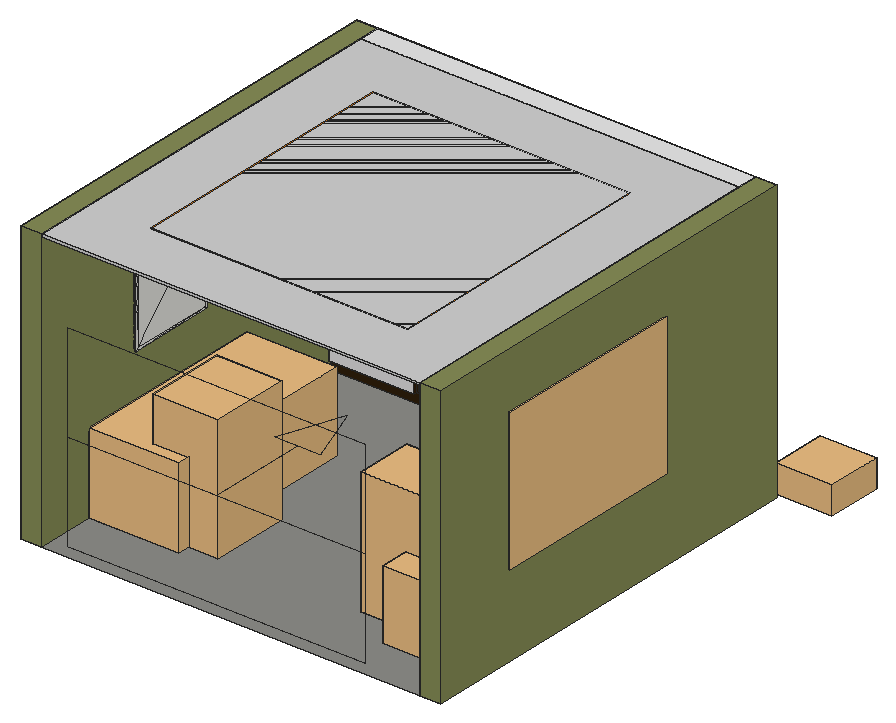
# SketchUp Ruby script. Lengths in inches.
U = 1.inch
M = Sketchup.active_model
def pt(a) = Geom::Point3d.new(a.map { |v| v * U })
def face(e, loops, mat)
  f = e.add_face(loops[0].map { |a| pt(a) })
  loops[1..].each { |l| e.add_face(l.map { |a| pt(a) }).erase! }
  f.material = f.back_material = mat if mat
  f
end
# faces: each face lists its corners as indices into pts; further lists are holes
def faces(e, pts, list, mat = nil) = list.each { |f| face(e, (f[0].is_a?(Array) ? f : [f]).map { |l| l.map { |i| pts[i] } }, mat) }
# xy, xz, yz: faces in a plane at the given z, y or x. An outline is a flat list of corners, or four numbers for a rectangle; further outlines are holes
def ring(l) = l.size == 4 ? [[l[0], l[1]], [l[2], l[1]], [l[2], l[3]], [l[0], l[3]]] : l.each_slice(2).to_a
def flat(e, list, mat, &to3) = list.each { |f| face(e, (f[0].is_a?(Array) ? f : [f]).map { |l| ring(l).map { |u, v| to3.(u, v) } }, mat) }
def xy(e, z, list, mat = nil) = flat(e, list, mat) { |x, y| [x, y, z] }
def xz(e, y, list, mat = nil) = flat(e, list, mat) { |x, z| [x, y, z] }
def yz(e, x, list, mat = nil) = flat(e, list, mat) { |y, z| [x, y, z] }
def lines(e, pts, list) = list.each { |a, b| e.add_line(pt(pts[a]), pt(pts[b])) }
# prism: a flat outline (further loops are holes) pulled along v
def prism(e, loops, v, mat = nil)
  f = face(e, loops, mat); d = Geom::Vector3d.new(v.map { |x| x * U })
  f.pushpull(f.normal.samedirection?(d) ? d.length : -d.length)
end
def box(e, o, s, mat = nil) = prism(e, [[o, [o[0] + s[0], o[1], o[2]], [o[0] + s[0], o[1] + s[1], o[2]], [o[0], o[1] + s[1], o[2]]]], [0, 0, s[2]], mat)
def at(x, y, z, deg = 0) = Geom::Transformation.translation(pt([x, y, z])) * Geom::Transformation.rotation(ORIGIN, Z_AXIS, deg.degrees)
def axes(o, x, y, z) = Geom::Transformation.new([*x, 0, *y, 0, *z, 0, *pt(o).to_a, 1])
def part(name) = M.definitions.add(name)
# library, detail: a bought-in or finely detailed component or shape, given as its bounding box
def library(name, o, s) = part(name).tap { |d| box(d.entities, o, s) }
def detail(e, o, s) = box(e.add_group.entities, o, s)
def put(e, d, t, mat = nil) = e.add_instance(d, t).tap { |i| i.material = mat if mat }
def group(e, t, mat = nil) = e.add_group.tap { |g| g.transformation = t; g.material = mat if mat }.entities
root = M.entities
M.materials.add("Emissive").color = [255, 146, 33]
M.materials.add("Emissive\#1").color = [255, 146, 33]
M.materials.add("Marble White 23-73 150cm").color = [221, 220, 222]
M.materials.add("Marble White SSS 100cm").color = [222, 222, 222]
M.materials.add("Tiles Grey 13 135cm").color = [141, 141, 136]
M.materials.add("Wall Paint Fine Grain 01 White 100cm").color = [208, 208, 208]
M.materials.add("Wall Paint Olive Matte 300cm").color = [133, 140, 86]
M.materials.add("Wall Paint White Semigloss 300cm").color = [232, 232, 232]
M.materials.add("Wood Walnut 33-38 100cm").color = [48, 31, 12]
c1 = library("Rue De Babylone Sofa",[-49.17,-15.95,0],[98.34,31.9,29.73])
c2 = library("Vera Sofa with Skirt",[-42.23,-17.43,0],[84.46,38.26,34.375])
c3 = library("Books 284 012",[-3.9,-5.03,0],[7.8,10.06,1.71])
c4 = library("Radio 114 011",[-4.52,-2.59,0],[9.04,5.18,10])
c5 = library("Metal Robot 114 042",[-2.05,-1.33,0],[4.11,2.66,7.35])
c6 = library("Interior Props 221 021",[-4.05,-2.74,-0.04],[8.1,5.5,13.08])
c7 = library("Vase 193 006",[-6.57,-6.63,0],[14.76,12.62,17.43])
c8 = library("Magazine 193 001",[-10.16,-7.05,0],[21.59,13.95,2.71])
c9 = library("Vase 004",[-7.23,-6.39,-0.02],[13.74,12.68,17.81])
c10 = library("Router 156 006",[-4.3,-2.49,-0.03],[9,4.96,4.68])
c11 = library("Toy 155 013",[-1.73,-1.4375,0],[3.14,2.99,4.15])
c12 = part("Print Art 008")
xy(c12.entities,-18.54,[[-18.4,-0.29,-18.4,-0.1,18.4,-0.29],[18.4,-0.29,-18.4,-0.1,18.4,-0.1]])
xy(c12.entities,-18.02,[[-18.02,-0.98,18.02,-0.01,-18.02,-0.01],[-18.02,-0.98,18.02,-0.98,18.02,-0.01]])
xy(c12.entities,-18,[[-18,-0.94,-18,-0.45,18,-0.94],[18,-0.94,-18,-0.45,18,-0.45]])
xy(c12.entities,18,[[-18,-0.94,18,-0.45,-18,-0.45],[-18,-0.94,18,-0.94,18,-0.45]])
xy(c12.entities,18.02,[[-18.02,-0.98,-18.02,-0.01,18.02,-0.98],[18.02,-0.98,-18.02,-0.01,18.02,-0.01]])
xy(c12.entities,18.54,[[-18.4,-0.29,18.4,-0.1,-18.4,-0.1],[-18.4,-0.29,18.4,-0.29,18.4,-0.1]])
xz(c12.entities,-0.98,[[-18.99,-18.99,-18.02,-18.02,-18.99,18.99],[-18.99,-18.99,18.02,-18.02,-18.02,-18.02],[-18.99,-18.99,18.99,-18.99,18.02,-18.02],[18.99,-18.99,18.02,18.02,18.02,-18.02],[18.99,-18.99,18.99,18.99,18.02,18.02],
  [-18.02,-18.02,-18.02,18.02,-18.99,18.99],[-18.02,18.02,18.99,18.99,-18.99,18.99],[-18.02,18.02,18.02,18.02,18.99,18.99]])
xz(c12.entities,-0.94,[[-18,-18,18,-18,18,18],[-18,-18,18,18,-18,18]])
xz(c12.entities,-0.45,[[-18,-18,-18,18,18,18],[-18,-18,18,18,18,-18]])
xz(c12.entities,-0.29,[[-18.4,-18.54,18.4,-18.54,18.4,18.54],[-18.4,-18.54,18.4,18.54,-18.4,18.54]])
xz(c12.entities,-0.1,[[-18.4,-18.54,-18.4,18.54,18.4,18.54],[-18.4,-18.54,18.4,18.54,18.4,-18.54]])
xz(c12.entities,-0.01,[[-18.98,-18.98,-18.02,-18.02,18.98,-18.98],[-18.98,-18.98,-18.02,18.02,-18.02,-18.02],[-18.98,-18.98,-18.98,18.98,-18.02,18.02],[18.98,-18.98,-18.02,-18.02,18.02,-18.02],[18.98,-18.98,18.02,-18.02,18.98,18.98],
  [18.02,-18.02,18.02,18.02,18.98,18.98],[-18.02,18.02,-18.98,18.98,18.02,18.02],[18.02,18.02,-18.98,18.98,18.98,18.98]])
yz(c12.entities,-18.4,[[-0.29,-18.54,-0.1,18.54,-0.1,-18.54],[-0.29,-18.54,-0.29,18.54,-0.1,18.54]])
yz(c12.entities,-18.02,[[-0.01,-18.02,-0.01,18.02,-0.98,18.02],[-0.98,-18.02,-0.01,-18.02,-0.98,18.02]])
yz(c12.entities,-18,[[-0.94,-18,-0.45,18,-0.45,-18],[-0.94,-18,-0.94,18,-0.45,18]])
yz(c12.entities,18,[[-0.45,-18,-0.45,18,-0.94,18],[-0.94,-18,-0.45,-18,-0.94,18]])
yz(c12.entities,18.02,[[-0.98,-18.02,-0.01,18.02,-0.01,-18.02],[-0.98,-18.02,-0.98,18.02,-0.01,18.02]])
yz(c12.entities,18.4,[[-0.1,-18.54,-0.1,18.54,-0.29,18.54],[-0.29,-18.54,-0.1,-18.54,-0.29,18.54]])
p = [[-18.98,-0.01,18.98],[-18.98,-0.01,-18.98],[-18.99,-0.98,-18.99],[-18.99,-0.98,18.99],[18.98,-0.01,-18.98],[18.99,-0.98,-18.99],
  [18.98,-0.01,18.98],[18.99,-0.98,18.99]]
faces(c12.entities,p,[[0,1,2],[2,3,0],[1,4,5],[5,2,1],[4,6,7],[7,5,4],[6,0,3],[3,7,6]])
c13 = library("Air Conditioner 12-08",[-17.72,-4.75,-0.8125],[35.44,4.75,9.47])
c14 = library("Johnny Sitting 001",[-16.98,-13.88,0],[33.96,27.76,53.26])
c15 = library("Jerald Sitting 001",[-12.16,-14.11,0],[24.32,28.22,53.59])
c16 = part("Group37\#1")
p = [[0,0,0],[0,0,-6.8],[-2.75,0,-6.8],[17.875,-4.15,0],[-17.875,-4.15,0],[17.875,4.15,0],
  [17.875,0,0],[-17.875,4.15,0],[2.75,0,-6.8],[-17.875,0,0],[0,0,-11.01]]
lines(c16.entities,p,[[0,1],[1,2],[3,4],[5,6],[7,5],[1,8],[9,0],[0,6],[8,10],[4,9],[6,3],[2,10],
  [9,7]])
c17 = part("Rectangle Light")
put(c17.entities,c16,at(0,0,0))
c18 = library("IES Light",[-4.45,-4.45,-12],[8.9,8.9,12])
c19 = library("Dome Light",[-12,-12,0],[24,24,12])
c20 = part("Group45\#1")
p = [[0,0,0],[0,0,-43.4],[-12.44,0,-43.4],[81,-59.5,0],[-81,-59.5,0],[81,59.5,0],
  [81,0,0],[-81,59.5,0],[12.44,0,-43.4],[-81,0,0],[0,0,-70.25]]
lines(c20.entities,p,[[0,1],[1,2],[3,4],[5,6],[7,5],[1,8],[9,0],[0,6],[8,10],[4,9],[6,3],[2,10],
  [9,7]])
c21 = part("Rectangle Light\#1")
put(c21.entities,c20,at(0,0,0))
c22 = library("Curtains 47-25 merged",[-45.98,-3.97,-0.23],[91.96,10.81,94.58])
c23 = library("Window 46-08 merged",[-34.875,-3.16,0],[69.74,4.26,70.87])
c24 = library("TV 156 039 merged",[-24.43,-3.69,-0.14],[48.87,7.6,29.26])
c25 = part("Vertical wall slat")
xy(c25.entities,-47.05,[[195.61,-2,197.61,0]])
xy(c25.entities,60.95,[[195.61,-2,197.61,0]])
xz(c25.entities,-2,[[195.61,-47.05,197.61,60.95]],"Wood Walnut 33-38 100cm")
xz(c25.entities,0,[[195.61,-47.05,197.61,60.95]])
yz(c25.entities,195.61,[[-2,-47.05,0,60.95]])
yz(c25.entities,197.61,[[-2,-47.05,0,60.95]],"Wood Walnut 33-38 100cm")
c26 = library("IES Light\#1",[-4.45,-4.45,-12],[8.9,8.9,12])
c27 = part("Recessed downlight")
xy(c27.entities,-1,[[3,1,3.52,1.07,4,1.27,4.41,1.59,4.73,2,4.93,2.48,5,3,4.93,3.52,4.73,4,4.41,4.41,4,4.73,3.52,4.93,3,5,2.48,4.93,2,4.73,1.59,4.41,1.27,4,1.07,3.52,1,3,1.07,2.48,1.27,2,1.59,1.59,2,1.27,2.48,1.07]])
xy(c27.entities,0,[[[3,0,2.22,0.1,1.5,0.4,0.88,0.88,0.4,1.5,0.1,2.22,0,3,0.1,3.78,0.4,4.5,0.88,5.12,1.5,5.6,2.22,5.9,3,6,3.78,5.9,4.5,5.6,5.12,5.12,5.6,4.5,5.9,3.78,6,3,5.9,2.22,5.6,1.5,5.12,0.88,4.5,0.4,3.78,0.1],[3,1,3.52,1.07,4,1.27,4.41,1.59,4.73,2,4.93,2.48,5,3,4.93,3.52,4.73,4,4.41,4.41,4,4.73,3.52,4.93,3,5,2.48,4.93,2,4.73,1.59,4.41,1.27,4,1.07,3.52,1,3,1.07,2.48,1.27,2,1.59,1.59,2,1.27,2.48,1.07]]])
xy(c27.entities,0.5,[[[3,0,3.78,0.1,4.5,0.4,5.12,0.88,5.6,1.5,5.9,2.22,6,3,5.9,3.78,5.6,4.5,5.12,5.12,4.5,5.6,3.78,5.9,3,6,2.22,5.9,1.5,5.6,0.88,5.12,0.4,4.5,0.1,3.78,0,3,0.1,2.22,0.4,1.5,0.88,0.88,1.5,0.4,2.22,0.1],[3,1,2.48,1.07,2,1.27,1.59,1.59,1.27,2,1.07,2.48,1,3,1.07,3.52,1.27,4,1.59,4.41,2,4.73,2.48,4.93,3,5,3.52,4.93,4,4.73,4.41,4.41,4.73,4,4.93,3.52,5,3,4.93,2.48,4.73,2,4.41,1.59,4,1.27,3.52,1.07]]])
p = [[2.48,1.07,-1],[2.48,1.07,0],[2.48,1.07,0.5],[3,1,0.5],[3,1,0],[3,1,-1],
  [3.52,1.07,0.5],[3.52,1.07,0],[3.52,1.07,-1],[2,1.27,-1],[2,1.27,0],[2,1.27,0.5],
  [4,1.27,0.5],[4,1.27,0],[4,1.27,-1],[1.59,1.59,-1],[1.59,1.59,0],[1.59,1.59,0.5],
  [4.41,1.59,0.5],[4.41,1.59,0],[4.41,1.59,-1],[1.27,2,-1],[1.27,2,0],[1.27,2,0.5],
  [4.73,2,0.5],[4.73,2,0],[4.73,2,-1],[1.07,2.48,-1],[1.07,2.48,0],[1.07,2.48,0.5],
  [4.93,2.48,0.5],[4.93,2.48,0],[4.93,2.48,-1],[1,3,-1],[1,3,0],[1,3,0.5],
  [5,3,0.5],[5,3,0],[5,3,-1],[1.07,3.52,-1],[1.07,3.52,0],[1.07,3.52,0.5],
  [4.93,3.52,0.5],[4.93,3.52,0],[4.93,3.52,-1],[1.27,4,-1],[1.27,4,0],[1.27,4,0.5],
  [4.73,4,0.5],[4.73,4,0],[4.73,4,-1],[1.59,4.41,-1],[1.59,4.41,0],[1.59,4.41,0.5],
  [4.41,4.41,0.5],[4.41,4.41,0],[4.41,4.41,-1],[2,4.73,-1],[2,4.73,0],[2,4.73,0.5],
  [4,4.73,0.5],[4,4.73,0],[4,4.73,-1],[2.48,4.93,-1],[2.48,4.93,0],[2.48,4.93,0.5],
  [3.52,4.93,0.5],[3.52,4.93,0],[3.52,4.93,-1],[3,5,-1],[3,5,0],[3,5,0.5],
  [2.22,0.1,0],[3,0,0],[3,0,0.5],[2.22,0.1,0.5],[3.78,0.1,0],[3.78,0.1,0.5],
  [1.5,0.4,0],[1.5,0.4,0.5],[4.5,0.4,0],[4.5,0.4,0.5],[0.88,0.88,0],[0.88,0.88,0.5],
  [5.12,0.88,0],[5.12,0.88,0.5],[0.4,1.5,0],[0.4,1.5,0.5],[5.6,1.5,0],[5.6,1.5,0.5],
  [0.1,2.22,0],[0.1,2.22,0.5],[5.9,2.22,0],[5.9,2.22,0.5],[0,3,0],[0,3,0.5],
  [6,3,0],[6,3,0.5],[0.1,3.78,0],[0.1,3.78,0.5],[5.9,3.78,0],[5.9,3.78,0.5],
  [0.4,4.5,0],[0.4,4.5,0.5],[5.6,4.5,0],[5.6,4.5,0.5],[0.88,5.12,0],[0.88,5.12,0.5],
  [5.12,5.12,0],[5.12,5.12,0.5],[1.5,5.6,0],[1.5,5.6,0.5],[4.5,5.6,0],[4.5,5.6,0.5],
  [2.22,5.9,0],[2.22,5.9,0.5],[3.78,5.9,0],[3.78,5.9,0.5],[3,6,0],[3,6,0.5]]
faces(c27.entities,p,[[0,1,2,3,4,5],[5,4,3,6,7,8],[9,10,11,2,1,0],[8,7,6,12,13,14],[15,16,17,11,10,9],[14,13,12,18,19,20],[21,22,23,17,16,15],[20,19,18,24,25,26],
  [27,28,29,23,22,21],[26,25,24,30,31,32],[33,34,35,29,28,27],[32,31,30,36,37,38],[39,40,41,35,34,33],[38,37,36,42,43,44],[45,46,47,41,40,39],[44,43,42,48,49,50],
  [51,52,53,47,46,45],[50,49,48,54,55,56],[57,58,59,53,52,51],[56,55,54,60,61,62],[63,64,65,59,58,57],[62,61,60,66,67,68],[69,70,71,65,64,63],[68,67,66,71,70,69],
  [72,73,74,75],[73,76,77,74],[78,72,75,79],[76,80,81,77],[82,78,79,83],[80,84,85,81],[86,82,83,87],[84,88,89,85],
  [90,86,87,91],[88,92,93,89],[94,90,91,95],[92,96,97,93],[98,94,95,99],[96,100,101,97],[102,98,99,103],[100,104,105,101],
  [106,102,103,107],[104,108,109,105],[110,106,107,111],[108,112,113,109],[114,110,111,115],[112,116,117,113],[118,114,115,119],[116,118,119,117]])
put(c27.entities,c26,axes([3,3,0.76],[1,0,0],[0,1,0],[0,0,-1]))
xy(root,47.32,[[61.2,168.17,60.93,168.26,61.48,168.22],[82.18,168.17,81.91,168.26,82.46,168.22],[61.48,168.22,60.93,168.26,61.78,168.68],[61.48,168.22,61.78,168.68,61.69,168.41],[82.46,168.22,81.91,168.26,82.76,168.68],
  [82.46,168.22,82.76,168.68,82.67,168.41],[60.93,168.26,60.69,168.75,60.99,169.21],[60.93,168.26,60.74,168.47,60.69,168.75],[60.93,168.26,60.99,169.21,61.78,168.68],[81.91,168.26,81.66,168.75,81.97,169.21],
  [81.91,168.26,81.72,168.47,81.66,168.75],[81.91,168.26,81.97,169.21,82.76,168.68],[61.78,168.68,60.99,169.21,61.54,169.17],[61.78,168.68,61.54,169.17,61.73,168.96],[82.76,168.68,81.97,169.21,82.52,169.17],
  [82.76,168.68,82.52,169.17,82.71,168.96],[60.69,168.75,60.78,169.02,60.99,169.21],[81.66,168.75,81.76,169.02,81.97,169.21],[61.54,169.17,60.99,169.21,61.27,169.26],[82.52,169.17,81.97,169.21,82.25,169.26]])
xy(root,47.36,[[61.2,168.17,61.48,168.22,60.93,168.26],[82.18,168.17,82.46,168.22,81.91,168.26],[61.48,168.22,60.69,168.75,60.93,168.26],[61.48,168.22,61.54,169.17,60.69,168.75],[61.48,168.22,61.69,168.41,61.78,168.68],
  [61.48,168.22,61.78,168.68,61.54,169.17],[82.46,168.22,81.66,168.75,81.91,168.26],[82.46,168.22,82.52,169.17,81.66,168.75],[82.46,168.22,82.67,168.41,82.76,168.68],[82.46,168.22,82.76,168.68,82.52,169.17],
  [60.93,168.26,60.69,168.75,60.74,168.47],[81.91,168.26,81.66,168.75,81.72,168.47],[61.78,168.68,61.73,168.96,61.54,169.17],[82.76,168.68,82.71,168.96,82.52,169.17],[60.69,168.75,60.99,169.21,60.78,169.02],
  [60.69,168.75,61.54,169.17,60.99,169.21],[81.66,168.75,81.97,169.21,81.76,169.02],[81.66,168.75,82.52,169.17,81.97,169.21],[61.54,169.17,61.27,169.26,60.99,169.21],[82.52,169.17,82.25,169.26,81.97,169.21]])
p = [[61.2,168.17,47.36],[60.93,168.26,47.36],[60.93,168.26,47.32],[61.2,168.17,47.32],[61.48,168.22,47.36],[61.48,168.22,47.32],
  [61.69,168.41,47.36],[61.69,168.41,47.32],[82.18,168.17,47.36],[81.91,168.26,47.36],[81.91,168.26,47.32],[82.18,168.17,47.32],
  [82.46,168.22,47.36],[82.46,168.22,47.32],[82.67,168.41,47.36],[82.67,168.41,47.32],[60.74,168.47,47.36],[60.74,168.47,47.32],
  [81.72,168.47,47.36],[81.72,168.47,47.32],[61.78,168.68,47.36],[61.78,168.68,47.32],[82.76,168.68,47.36],[82.76,168.68,47.32],
  [60.69,168.75,47.36],[60.69,168.75,47.32],[81.66,168.75,47.36],[81.66,168.75,47.32],[61.73,168.96,47.36],[61.73,168.96,47.32],
  [82.71,168.96,47.36],[82.71,168.96,47.32],[60.78,169.02,47.36],[60.78,169.02,47.32],[81.76,169.02,47.36],[81.76,169.02,47.32],
  [60.99,169.21,47.36],[60.99,169.21,47.32],[61.54,169.17,47.36],[61.54,169.17,47.32],[81.97,169.21,47.36],[81.97,169.21,47.32],
  [82.52,169.17,47.36],[82.52,169.17,47.32],[61.27,169.26,47.36],[61.27,169.26,47.32],[82.25,169.26,47.36],[82.25,169.26,47.32]]
faces(root,p,[[0,1,2],[2,3,0],[4,0,3],[3,5,4],[6,4,5],[5,7,6],[8,9,10],[10,11,8],
  [12,8,11],[11,13,12],[14,12,13],[13,15,14],[1,16,17],[17,2,1],[9,18,19],[19,10,9],
  [20,6,7],[7,21,20],[22,14,15],[15,23,22],[16,24,25],[25,17,16],[18,26,27],[27,19,18],
  [28,20,21],[21,29,28],[30,22,23],[23,31,30],[24,32,33],[33,25,24],[26,34,35],[35,27,26],
  [32,36,37],[37,33,32],[38,28,29],[29,39,38],[34,40,41],[41,35,34],[42,30,31],[31,43,42],
  [36,44,45],[45,37,36],[44,38,39],[39,45,44],[40,46,47],[47,41,40],[46,42,43],[43,47,46]])
put(root,c1,axes([155.05,69.1875,0],[0,1,0],[1,0,0],[0,0,1]))
put(root,c2,at(29.83,67.89,0,90))
put(root,c3,at(100.82,160.36,10))
put(root,c3,at(18.98,161.07,16))
put(root,c3,at(164.75,160.875,88.65))
put(root,c4,at(165.17,161.59,18.67))
put(root,c4,at(112.48,159.44,16))
put(root,c5,at(164.75,157,54.32))
put(root,c5,at(28.22,159,16))
put(root,c6,at(153.25,159.74,79.57))
put(root,c6,at(101.77,159.46,16))
put(root,c7,at(63.52,161.36,16))
put(root,c8,at(151.35,99.1,15.21))
put(root,c8,at(35.08,89.79,19.11))
put(root,c9,axes([153.52,163.39,53.02],[0.76413,0,0],[0,1,0],[0,0,1]))
put(root,c9,axes([153.52,160.4375,27.27],[0.76413,0,0],[0,1,0],[0,0,1]))
put(root,c9,axes([153.52,159,1.35],[0.76413,0,0],[0,1,0],[0,0,1]))
put(root,c3,at(164.92,162.66,35.79))
put(root,c10,at(43.27,160.02,16))
put(root,c11,at(164.87,159.84,70.17))
put(root,c12,at(8.99,68.5625,72.53,90))
put(root,c13,at(9,116.47,87.12,90))
put(root,c14,at(46.07,47.85,0,90))
put(root,c15,at(134.01,44.68,0,-90))
put(root,c17,axes([27.75,159.85,14.49],[1,0,0],[0,-1,0],[0,0,0.36]))
put(root,c17,axes([65.84,159.85,14.49],[1,0,0],[0,-1,0],[0,0,0.36]))
put(root,c17,axes([103.33,159.85,14.49],[0.89884,0,0],[0,-1,0],[0,0,0.36]))
put(root,c17,axes([63,161.85,8.25],[0.8633,0,0],[0,-1,0],[0,0,0.22453]))
put(root,c18,axes([153.25,162.05,103.49],[1,0,0],[0,1,0],[0,0,0.78]))
put(root,c18,axes([164.91,162.05,103.49],[1,0,0],[0,1,0],[0,0,0.78]))
put(root,c18,axes([164.91,162.05,85.5625],[1,0,0],[0,1,0],[0,0,0.78]))
put(root,c18,axes([164.91,162.05,67.81],[1,0,0],[0,1,0],[0,0,0.78]))
put(root,c18,axes([153.25,162.05,76.89],[1,0,0],[0,1,0],[0,0,0.78]))
put(root,c18,axes([153.25,162.05,50.99],[1,0,0],[0,1,0],[0,0,0.78]))
put(root,c18,axes([153.25,162.05,25.07],[1,0,0],[0,1,0],[0,0,0.78]))
put(root,c18,axes([164.91,162.05,50.4],[1,0,0],[0,1,0],[0,0,0.78]))
put(root,c18,axes([164.91,162.05,32.99],[1,0,0],[0,1,0],[0,0,0.78]))
put(root,c18,axes([164.91,162.05,15.58],[1,0,0],[0,1,0],[0,0,0.78]))
put(root,c19,at(190.13,193.56,0))
put(root,c21,axes([90.51,-8.13,52.01],[0.7863,0,0],[0,0,-0.70597],[0,-1,0]))
put(root,c22,axes([164.16,79.1,32.65],[0,-1.2932,0],[1,0,0],[0,0,0.7663]))
put(root,c23,axes([176,78,36],[0,1.20437,0],[-1.5872,0,0],[0,0,0.84667]))
put(root,c24,at(73.52,161.09,48.2))
g1 = group(root,at(0,0,0),"Tiles Grey 13 135cm")
xy(g1,0,[[0,0,180,180]],"Tiles Grey 13 135cm")
g2 = group(root,at(0,0,0),"Wall Paint Olive Matte 300cm")
box(g2,[0,0,0],[9,180,120])
g3 = group(root,at(171,0,0),"Wall Paint Olive Matte 300cm")
prism(g3,[[[9,0,0],[9,180,0],[9,180,120],[9,0,120]],[[9,120,96],[9,120,36],[9,36,36],[9,36,96]]],[-9,0,0])
g4 = group(root,at(9,171,0),"Wall Paint White Semigloss 300cm")
box(g4,[0,0,0],[162,9,120])
g5 = group(root,at(9,169,0),"Marble White SSS 100cm")
box(g5,[0,0,0],[162,2,108],"Marble White SSS 100cm")
g6 = group(root,at(147,157,0),"Wood Walnut 33-38 100cm")
xy(g6,0,[[0,0,24,12]],"Wood Walnut 33-38 100cm")
xy(g6,1,[[1,0,11.5,10],[12.5,0,23,10]],"Wood Walnut 33-38 100cm")
xy(g6,17.67,[[12.5,0,23,10]],"Wood Walnut 33-38 100cm")
xy(g6,18.67,[[12.5,0,23,10]],"Wood Walnut 33-38 100cm")
xy(g6,26.25,[[1,0,11.5,10]],"Wood Walnut 33-38 100cm")
xy(g6,27.25,[[1,0,11.5,10]],"Wood Walnut 33-38 100cm")
xy(g6,34.83,[[12.5,0,23,10]],"Wood Walnut 33-38 100cm")
xy(g6,35.83,[[12.5,0,23,10]],"Wood Walnut 33-38 100cm")
xy(g6,52,[[1,0,11.5,10],[12.5,0,23,10]],"Wood Walnut 33-38 100cm")
xy(g6,53,[[1,0,11.5,10],[12.5,0,23,10]],"Wood Walnut 33-38 100cm")
xy(g6,69.17,[[12.5,0,23,10]],"Wood Walnut 33-38 100cm")
xy(g6,70.17,[[12.5,0,23,10]],"Wood Walnut 33-38 100cm")
xy(g6,77.75,[[1,0,11.5,10]],"Wood Walnut 33-38 100cm")
xy(g6,78.75,[[1,0,11.5,10]],"Wood Walnut 33-38 100cm")
xy(g6,86.33,[[12.5,0,23,10]],"Wood Walnut 33-38 100cm")
xy(g6,87.33,[[12.5,0,23,10]],"Wood Walnut 33-38 100cm")
xy(g6,104,[[1,0,11.5,10],[12.5,0,23,10]],"Wood Walnut 33-38 100cm")
xy(g6,108,[[0,0,24,12]],"Wood Walnut 33-38 100cm")
xz(g6,0,[[[0,0,24,108],[1,78.75,11.5,104],[1,1,11.5,26.25],[1,53,11.5,77.75],[1,27.25,11.5,52],[12.5,1,23,17.67],[12.5,87.33,23,104],[12.5,70.17,23,86.33],[12.5,35.83,23,52],[12.5,53,23,69.17],[12.5,18.67,23,34.83]]],"Wood Walnut 33-38 100cm")
xz(g6,10,[[1,1,11.5,26.25],[12.5,1,23,17.67],[12.5,18.67,23,34.83],[1,27.25,11.5,52],[12.5,35.83,23,52],
  [1,53,11.5,77.75],[12.5,53,23,69.17],[12.5,70.17,23,86.33],[1,78.75,11.5,104],[12.5,87.33,23,104]],"Wood Walnut 33-38 100cm")
xz(g6,12,[[0,0,24,108]],"Wood Walnut 33-38 100cm")
yz(g6,0,[[0,0,12,108]],"Wood Walnut 33-38 100cm")
yz(g6,1,[[0,1,10,26.25],[0,27.25,10,52],[0,53,10,77.75],[0,78.75,10,104]],"Wood Walnut 33-38 100cm")
yz(g6,11.5,[[0,1,10,26.25],[0,27.25,10,52],[0,53,10,77.75],[0,78.75,10,104]],"Wood Walnut 33-38 100cm")
yz(g6,12.5,[[0,1,10,17.67],[0,18.67,10,34.83],[0,35.83,10,52],[0,53,10,69.17],[0,70.17,10,86.33],
  [0,87.33,10,104]],"Wood Walnut 33-38 100cm")
yz(g6,23,[[0,1,10,17.67],[0,18.67,10,34.83],[0,35.83,10,52],[0,53,10,69.17],[0,70.17,10,86.33],
  [0,87.33,10,104]],"Wood Walnut 33-38 100cm")
yz(g6,24,[[0,0,12,108]],"Wood Walnut 33-38 100cm")
g7 = group(root,at(9,154,0))
xy(g7,0,[[0,1,114,13]],"Wood Walnut 33-38 100cm")
xy(g7,4,[[0,0,36.5,1],[71.5,0,108,1],[0,1,0,13,114,13,114,1,113,1,113,12,108,12,108,1],[108,1,113,12]],"Wood Walnut 33-38 100cm")
xy(g7,5,[[37.5,1,70.5,12]],"Wood Walnut 33-38 100cm")
xy(g7,9,[[37.5,1,38.5,12],[38.5,1,70.5,12]],"Wood Walnut 33-38 100cm")
xy(g7,10,[[0,0,36.5,1],[71.5,0,75.5,1],[75.5,0,76.5,1],[76.5,0,108,1],[0,1,37.5,12],
  [38.5,1,75.5,12],[76.5,1,108,12]],"Wood Walnut 33-38 100cm")
xy(g7,15,[[0,1,37.5,12],[38.5,1,75.5,12],[76.5,1,113,12]],"Wood Walnut 33-38 100cm")
xy(g7,16,[[0,1,114,13]],"Wood Walnut 33-38 100cm")
xz(g7,1,[[0,0,114,4],[0,4,36.5,10],[113,4,114,4,114,16,0,16,0,15,37.5,15,37.5,10,38.5,10,38.5,15,75.5,15,75.5,10,76.5,10,76.5,15,113,15],[[36.5,4,71.5,10],[37.5,5,70.5,9]],[71.5,4,108,10]],"Wood Walnut 33-38 100cm")
xz(g7,12,[[108,4,113,4,113,15,76.5,15,76.5,10,108,10],[37.5,5,70.5,9],[0,10,37.5,15],[38.5,10,75.5,15]],"Wood Walnut 33-38 100cm")
xz(g7,13,[[0,0,114,4],[0,4,114,10],[0,10,114,16]],"Wood Walnut 33-38 100cm")
yz(g7,0,[[1,0,13,4],[0,4,1,10],[1,4,13,10],[12,10,12,15,1,15,1,16,13,16,13,10]],"Wood Walnut 33-38 100cm")
yz(g7,36.5,[[0,4,1,10]],"Wood Walnut 33-38 100cm")
yz(g7,37.5,[[1,5,12,9],[1,10,12,15]],"Wood Walnut 33-38 100cm")
yz(g7,38.5,[[1,10,12,15]],"Wood Walnut 33-38 100cm")
yz(g7,70.5,[[1,5,12,9]],"Wood Walnut 33-38 100cm")
yz(g7,71.5,[[0,4,1,10]],"Wood Walnut 33-38 100cm")
yz(g7,75.5,[[1,10,12,15]],"Wood Walnut 33-38 100cm")
yz(g7,76.5,[[1,10,12,15]],"Wood Walnut 33-38 100cm")
yz(g7,108,[[0,4,1,10],[1,4,12,10]],"Wood Walnut 33-38 100cm")
yz(g7,113,[[1,4,12,15]],"Wood Walnut 33-38 100cm")
yz(g7,114,[[1,0,13,4],[1,4,13,10],[1,10,13,16]],"Wood Walnut 33-38 100cm")
g8 = group(g7,at(0,0,4),"Marble White 23-73 150cm")
xz(g8,0,[[0,0,36.5,6],[71.5,0,108,6]],"Marble White 23-73 150cm")
g9 = group(root,at(33,165,40),"Marble White 23-73 150cm")
xy(g9,0,[[0,0,78,2]],"Marble White 23-73 150cm")
xy(g9,2,[[2,2,76,4]],"Emissive")
xy(g9,42,[[2,2,76,4]],"Emissive")
xy(g9,44,[[0,0,78,2]],"Marble White 23-73 150cm")
xz(g9,0,[[0,0,78,44]],"Marble White 23-73 150cm")
xz(g9,2,[[0,0,2,42],[2,0,76,2],[76,0,78,42],[2,2,76,42],[0,42,78,44]],"Marble White 23-73 150cm")
xz(g9,4,[[2,2,76,42]],"Marble White 23-73 150cm")
yz(g9,0,[[0,0,2,44]],"Marble White 23-73 150cm")
yz(g9,2,[[2,2,4,42]],"Emissive")
yz(g9,76,[[2,2,4,42]],"Emissive")
yz(g9,78,[[0,0,2,44]],"Marble White 23-73 150cm")
g10 = group(root,at(81,167,0))
put(g10,c25,at(-135.875,2,47.05))
put(g10,c25,at(-157.21,2,47.05))
put(g10,c25,at(-178.54,2,47.05))
put(g10,c25,at(-161.47,2,47.05))
put(g10,c25,at(-174.27,2,47.05))
put(g10,c25,at(-131.61,2,47.05))
put(g10,c25,at(-187.07,2,47.05))
put(g10,c25,at(-152.94,2,47.05))
put(g10,c25,at(-170.01,2,47.05))
put(g10,c25,at(-195.61,2,47.05))
put(g10,c25,at(-191.34,2,47.05))
put(g10,c25,at(-165.74,2,47.05))
put(g10,c25,at(-148.67,2,47.05))
put(g10,c25,at(-144.41,2,47.05))
put(g10,c25,at(-140.14,2,47.05))
put(g10,c25,at(-182.81,2,47.05))
g11 = group(root,at(9,0,119))
put(g11,c27,axes([33,33,-4],[1,0,0],[0,1,0],[0,0,-1]),"Wall Paint Fine Grain 01 White 100cm")
put(g11,c27,axes([33,82.5,-4],[1,0,0],[0,1,0],[0,0,-1]),"Wall Paint Fine Grain 01 White 100cm")
put(g11,c27,axes([123,132,-4],[1,0,0],[0,1,0],[0,0,-1]),"Wall Paint Fine Grain 01 White 100cm")
put(g11,c27,axes([123,33,-4],[1,0,0],[0,1,0],[0,0,-1]),"Wall Paint Fine Grain 01 White 100cm")
put(g11,c27,axes([33,132,-4],[1,0,0],[0,1,0],[0,0,-1]),"Wall Paint Fine Grain 01 White 100cm")
put(g11,c27,axes([78,33,-4],[1,0,0],[0,1,0],[0,0,-1]),"Wall Paint Fine Grain 01 White 100cm")
put(g11,c27,axes([123,82.5,-4],[1,0,0],[0,1,0],[0,0,-1]),"Wall Paint Fine Grain 01 White 100cm")
put(g11,c27,axes([78,132,-4],[1,0,0],[0,1,0],[0,0,-1]),"Wall Paint Fine Grain 01 White 100cm")
g12 = group(g11,at(0,0,0),"Wall Paint Fine Grain 01 White 100cm")
box(g12,[0,0,0],[162,171,1])
g13 = group(g12,at(24,24,1))
g14 = group(g13,at(0,0,0))
xy(g14,-2,[[2,2,112,121]])
xy(g14,0,[[2,2,112,121]])
xz(g14,2,[[2,-2,112,0]],"Emissive\#1")
xz(g14,121,[[2,-2,112,0]],"Emissive\#1")
yz(g14,2,[[2,-2,121,0]],"Emissive\#1")
yz(g14,112,[[2,-2,121,0]],"Emissive\#1")
g15 = group(g13,at(0,0,-2))
box(g15,[0,0,-2],[114,123,2])
